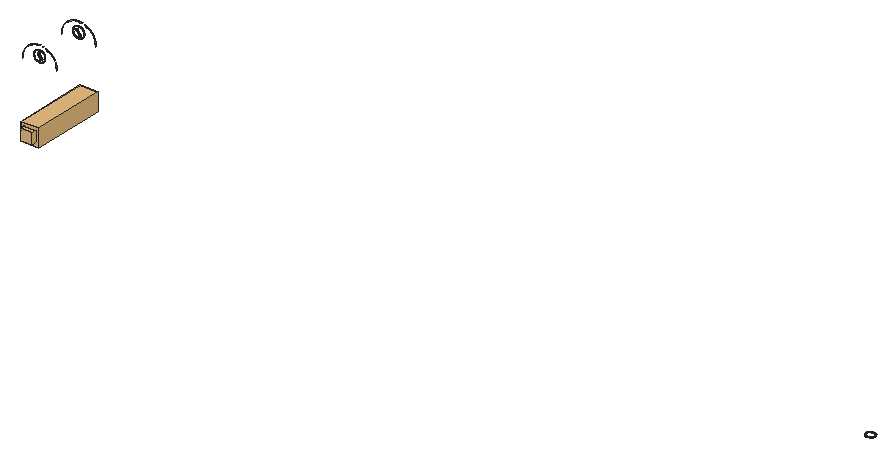
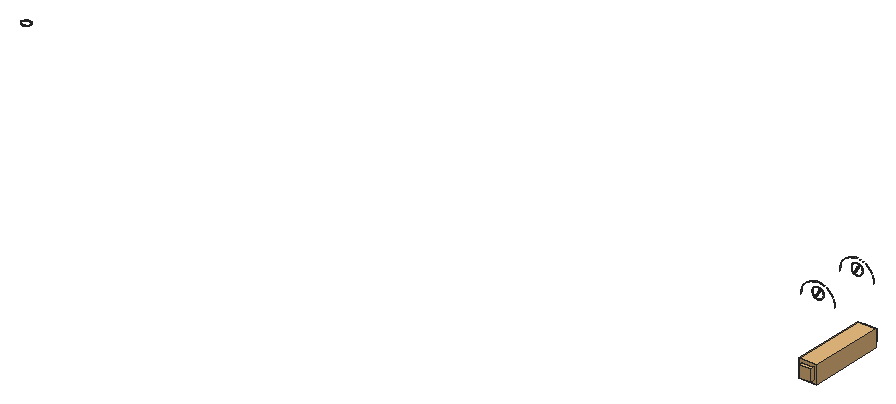
# SketchUp Ruby script. Lengths in inches.
U = 1.inch
M = Sketchup.active_model
def pt(a) = Geom::Point3d.new(a.map { |v| v * U })
def face(e, loops, mat)
  f = e.add_face(loops[0].map { |a| pt(a) })
  loops[1..].each { |l| e.add_face(l.map { |a| pt(a) }).erase! }
  f.material = f.back_material = mat if mat
  f
end
# faces: each face lists its corners as indices into pts; further lists are holes
def faces(e, pts, list, mat = nil) = list.each { |f| face(e, (f[0].is_a?(Array) ? f : [f]).map { |l| l.map { |i| pts[i] } }, mat) }
# xy, xz, yz: faces in a plane at the given z, y or x. An outline is a flat list of corners, or four numbers for a rectangle; further outlines are holes
def ring(l) = l.size == 4 ? [[l[0], l[1]], [l[2], l[1]], [l[2], l[3]], [l[0], l[3]]] : l.each_slice(2).to_a
def flat(e, list, mat, &to3) = list.each { |f| face(e, (f[0].is_a?(Array) ? f : [f]).map { |l| ring(l).map { |u, v| to3.(u, v) } }, mat) }
def xy(e, z, list, mat = nil) = flat(e, list, mat) { |x, y| [x, y, z] }
def xz(e, y, list, mat = nil) = flat(e, list, mat) { |x, z| [x, y, z] }
def yz(e, x, list, mat = nil) = flat(e, list, mat) { |y, z| [x, y, z] }
def lines(e, pts, list) = list.each { |a, b| e.add_line(pt(pts[a]), pt(pts[b])) }
# prism: a flat outline (further loops are holes) pulled along v
def prism(e, loops, v, mat = nil)
  f = face(e, loops, mat); d = Geom::Vector3d.new(v.map { |x| x * U })
  f.pushpull(f.normal.samedirection?(d) ? d.length : -d.length)
end
def box(e, o, s, mat = nil) = prism(e, [[o, [o[0] + s[0], o[1], o[2]], [o[0] + s[0], o[1] + s[1], o[2]], [o[0], o[1] + s[1], o[2]]]], [0, 0, s[2]], mat)
def at(x, y, z, deg = 0) = Geom::Transformation.translation(pt([x, y, z])) * Geom::Transformation.rotation(ORIGIN, Z_AXIS, deg.degrees)
def axes(o, x, y, z) = Geom::Transformation.new([*x, 0, *y, 0, *z, 0, *pt(o).to_a, 1])
def part(name) = M.definitions.add(name)
# library, detail: a bought-in or finely detailed component or shape, given as its bounding box
def library(name, o, s) = part(name).tap { |d| box(d.entities, o, s) }
def detail(e, o, s) = box(e.add_group.entities, o, s)
def put(e, d, t, mat = nil) = e.add_instance(d, t).tap { |i| i.material = mat if mat }
def group(e, t, mat = nil) = e.add_group.tap { |g| g.transformation = t; g.material = mat if mat }.entities
root = M.entities
M.materials.add("Material \#1").color = [140, 140, 140]
c1 = library("3DGeom~14_Defintion",[-102.17,352.37,-727.27],[204.35,204.35,1000])
c2 = library("3DGeom~1_Defintion",[-60.87,347.29,-704.08],[121.74,121.75,1000])
xy(root,193.77,[[371.53,115.15,371.46,115.17,371.53,115.17],[371.53,115.15,371.53,115.17,371.6,115.17],[371.53,115.15,371.6,115.17,371.6,115.15],[371.6,115.15,371.6,115.17,371.66,115.19],[371.6,115.15,371.66,115.19,371.67,115.17],
  [371.46,115.17,371.41,115.21,371.47,115.19],[371.46,115.17,371.47,115.19,371.53,115.17],[371.67,115.17,371.66,115.19,371.71,115.22],[371.67,115.17,371.71,115.22,371.72,115.21],[371.47,115.19,371.41,115.21,371.43,115.22],
  [371.41,115.21,371.375,115.26,371.43,115.22],[371.72,115.21,371.71,115.22,371.74,115.27],[371.72,115.21,371.74,115.27,371.76,115.26],[371.43,115.22,371.375,115.26,371.39,115.27],[371.375,115.26,371.36,115.32,371.39,115.27],
  [371.76,115.26,371.74,115.27,371.75,115.32],[371.76,115.26,371.75,115.32,371.77,115.32],[371.39,115.27,371.36,115.32,371.38,115.32],[371.36,115.32,371.375,115.38,371.38,115.32],[371.38,115.32,371.375,115.38,371.39,115.37],
  [371.75,115.32,371.74,115.37,371.77,115.32],[371.77,115.32,371.74,115.37,371.76,115.38],[371.39,115.37,371.375,115.38,371.41,115.43],[371.39,115.37,371.41,115.43,371.43,115.42],[371.74,115.37,371.71,115.42,371.76,115.38],
  [371.76,115.38,371.71,115.42,371.72,115.43],[371.43,115.42,371.41,115.43,371.46,115.47],[371.43,115.42,371.46,115.47,371.47,115.45],[371.71,115.42,371.66,115.45,371.72,115.43],[371.72,115.43,371.66,115.45,371.67,115.47],
  [371.47,115.45,371.46,115.47,371.53,115.49],[371.47,115.45,371.53,115.49,371.53,115.47],[371.66,115.45,371.6,115.47,371.67,115.47],[371.53,115.47,371.53,115.49,371.6,115.49],[371.53,115.47,371.6,115.49,371.6,115.47],
  [371.6,115.47,371.6,115.49,371.67,115.47]],"Material \#1")
xy(root,193.78,[[371.53,115.15,371.47,115.19,371.46,115.17],[371.53,115.15,371.53,115.17,371.47,115.19],[371.53,115.15,371.6,115.15,371.53,115.17],[371.6,115.15,371.6,115.17,371.53,115.17],[371.6,115.15,371.67,115.17,371.6,115.17],
  [371.46,115.17,371.43,115.22,371.41,115.21],[371.46,115.17,371.47,115.19,371.43,115.22],[371.6,115.17,371.67,115.17,371.66,115.19],[371.67,115.17,371.72,115.21,371.66,115.19],[371.66,115.19,371.72,115.21,371.71,115.22],
  [371.41,115.21,371.39,115.27,371.375,115.26],[371.41,115.21,371.43,115.22,371.39,115.27],[371.72,115.21,371.76,115.26,371.71,115.22],[371.71,115.22,371.76,115.26,371.74,115.27],[371.375,115.26,371.38,115.32,371.36,115.32],
  [371.375,115.26,371.39,115.27,371.38,115.32],[371.76,115.26,371.77,115.32,371.74,115.27],[371.74,115.27,371.77,115.32,371.75,115.32],[371.36,115.32,371.38,115.32,371.39,115.37],[371.36,115.32,371.39,115.37,371.375,115.38],
  [371.75,115.32,371.76,115.38,371.74,115.37],[371.75,115.32,371.77,115.32,371.76,115.38],[371.39,115.37,371.43,115.42,371.375,115.38],[371.74,115.37,371.72,115.43,371.71,115.42],[371.74,115.37,371.76,115.38,371.72,115.43],
  [371.375,115.38,371.43,115.42,371.41,115.43],[371.43,115.42,371.47,115.45,371.41,115.43],[371.71,115.42,371.67,115.47,371.66,115.45],[371.71,115.42,371.72,115.43,371.67,115.47],[371.41,115.43,371.47,115.45,371.46,115.47],
  [371.47,115.45,371.53,115.47,371.46,115.47],[371.66,115.45,371.6,115.49,371.6,115.47],[371.66,115.45,371.67,115.47,371.6,115.49],[371.46,115.47,371.53,115.47,371.53,115.49],[371.53,115.47,371.6,115.47,371.53,115.49],
  [371.6,115.47,371.6,115.49,371.53,115.49]],"Material \#1")
xz(root,114.63,[[337.35,195.92,337.36,196.05,337.36,195.92],[337.36,195.92,337.36,196.05,337.37,196.05],[338.75,195.92,338.74,196.05,338.77,195.92],[338.77,195.92,338.74,196.05,338.75,196.05],[338.06,195.97,338.01,195.98,338.06,195.99],
  [338.06,195.97,338.06,195.99,338.1,195.99],[338.06,195.97,338.1,195.99,338.1,195.98],[338.01,195.98,337.97,195.99,338.02,195.99],[338.01,195.98,338.02,195.99,338.06,195.99],[338.1,195.98,338.1,195.99,338.13,196],
  [338.1,195.98,338.13,196,338.14,195.99],[337.97,195.99,337.9375,196.01,337.98,196],[337.97,195.99,337.98,196,338.02,195.99],[338.14,195.99,338.13,196,338.17,196.02],[338.14,195.99,338.17,196.02,338.17,196.01],
  [337.98,196,337.9375,196.01,337.94,196.02],[337.9375,196.01,337.9,196.03,337.94,196.02],[338.17,196.01,338.17,196.02,338.2,196.04],[338.17,196.01,338.2,196.04,338.21,196.03],[337.94,196.02,337.9,196.03,337.91,196.04],
  [337.9,196.03,337.875,196.06,337.91,196.04],[338.21,196.03,338.2,196.04,338.23,196.0625],[338.21,196.03,338.23,196.0625,338.24,196.06],[337.91,196.04,337.875,196.06,337.88,196.0625],[337.36,196.05,337.39,196.17,337.37,196.05],
  [337.37,196.05,337.39,196.17,337.4,196.16],[338.74,196.05,338.71,196.16,338.75,196.05],[338.75,196.05,338.71,196.16,338.72,196.17],[337.875,196.06,337.85,196.09,337.88,196.0625],[338.24,196.06,338.23,196.0625,338.25,196.09],
  [338.24,196.06,338.25,196.09,338.26,196.09],[337.88,196.0625,337.85,196.09,337.86,196.09],[337.85,196.09,337.83,196.125,337.86,196.09],[337.86,196.09,337.83,196.125,337.85,196.13],[338.25,196.09,338.27,196.13,338.26,196.09],
  [338.26,196.09,338.27,196.13,338.28,196.125],[337.83,196.125,337.82,196.16,337.85,196.13],[338.28,196.125,338.27,196.13,338.28,196.16],[338.28,196.125,338.28,196.16,338.29,196.16],[337.85,196.13,337.82,196.16,337.84,196.16],
  [337.4,196.16,337.39,196.17,337.44,196.28],[337.4,196.16,337.44,196.28,337.45,196.27],[337.82,196.16,337.82,196.21,337.84,196.16],[337.84,196.16,337.82,196.21,337.83,196.21],[338.28,196.16,338.28,196.2,338.29,196.16],
  [338.29,196.16,338.28,196.2,338.29,196.2],[338.71,196.16,338.66,196.27,338.72,196.17],[338.72,196.17,338.66,196.27,338.67,196.28],[338.28,196.2,338.28,196.24,338.29,196.2],[338.29,196.2,338.28,196.24,338.29,196.24],
  [337.82,196.21,337.82,196.24,337.83,196.21],[337.83,196.21,337.82,196.24,337.84,196.24],[337.82,196.24,337.83,196.28,337.84,196.24],[337.84,196.24,337.83,196.28,337.85,196.28],[338.28,196.24,338.27,196.28,338.29,196.24],
  [338.29,196.24,338.27,196.28,338.28,196.28],[337.45,196.27,337.44,196.28,337.52,196.375],[337.45,196.27,337.52,196.375,337.52,196.37],[338.66,196.27,338.59,196.36,338.67,196.28],[337.83,196.28,337.85,196.32,337.85,196.28],
  [337.85,196.28,337.85,196.32,337.86,196.3125],[338.27,196.28,338.25,196.3125,338.28,196.28],[338.28,196.28,338.25,196.3125,338.26,196.32],[338.67,196.28,338.59,196.36,338.6,196.37],[337.86,196.3125,337.85,196.32,337.875,196.35],
  [337.86,196.3125,337.875,196.35,337.88,196.34],[338.25,196.3125,338.23,196.34,338.26,196.32],[338.26,196.32,338.23,196.34,338.24,196.35],[337.88,196.34,337.875,196.35,337.9,196.38],[337.88,196.34,337.9,196.38,337.91,196.37],
  [338.23,196.34,338.2,196.37,338.24,196.35],[338.24,196.35,338.2,196.37,338.21,196.38],[338.59,196.36,338.51,196.45,338.6,196.37],[337.52,196.37,337.52,196.375,337.6,196.46],[337.52,196.37,337.6,196.46,337.61,196.45],
  [337.91,196.37,337.9,196.38,337.9375,196.4],[337.91,196.37,337.9375,196.4,337.94,196.39],[338.2,196.37,338.17,196.39,338.21,196.38],[338.6,196.37,338.51,196.45,338.51,196.46],[338.21,196.38,338.17,196.39,338.17,196.4],
  [337.94,196.39,337.9375,196.4,337.97,196.42],[337.94,196.39,337.97,196.42,337.98,196.41],[338.17,196.39,338.13,196.41,338.17,196.4],[338.17,196.4,338.13,196.41,338.14,196.42],[337.98,196.41,337.97,196.42,338.01,196.43],
  [337.98,196.41,338.01,196.43,338.02,196.42],[338.13,196.41,338.1,196.42,338.14,196.42],[338.02,196.42,338.01,196.43,338.06,196.43],[338.02,196.42,338.06,196.43,338.06,196.42],[338.06,196.42,338.06,196.43,338.1,196.43],
  [338.06,196.42,338.1,196.43,338.1,196.42],[338.1,196.42,338.1,196.43,338.14,196.42],[337.61,196.45,337.6,196.46,337.7,196.52],[337.61,196.45,337.7,196.52,337.7,196.51],[338.51,196.45,338.41,196.51,338.51,196.46],
  [338.51,196.46,338.41,196.51,338.41,196.52],[337.7,196.51,337.7,196.52,337.81,196.57],[337.7,196.51,337.81,196.57,337.8125,196.5625],[338.41,196.51,338.3,196.5625,338.41,196.52],[338.41,196.52,338.3,196.5625,338.3,196.57],
  [337.8125,196.5625,337.81,196.57,337.93,196.61],[337.8125,196.5625,337.93,196.61,337.93,196.59],[338.3,196.5625,338.18,196.59,338.3,196.57],[338.3,196.57,338.18,196.59,338.18,196.61],[337.93,196.59,337.93,196.61,338.06,196.62],
  [337.93,196.59,338.06,196.62,338.06,196.61],[338.18,196.59,338.06,196.61,338.18,196.61],[338.06,196.61,338.06,196.62,338.18,196.61]],"Material \#1")
xz(root,116.63,[[337.35,195.92,337.36,195.92,337.36,196.05],[337.36,195.92,337.37,196.05,337.36,196.05],[338.75,195.92,338.77,195.92,338.74,196.05],[338.77,195.92,338.75,196.05,338.74,196.05],[338.06,195.97,338.06,195.99,338.01,195.98],
  [338.06,195.97,338.1,195.98,338.1,195.99],[338.06,195.97,338.1,195.99,338.06,195.99],[338.01,195.98,338.02,195.99,337.97,195.99],[338.01,195.98,338.06,195.99,338.02,195.99],[338.1,195.98,338.13,196,338.1,195.99],
  [338.1,195.98,338.14,195.99,338.13,196],[337.97,195.99,337.98,196,337.9375,196.01],[337.97,195.99,338.02,195.99,337.98,196],[338.14,195.99,338.17,196.02,338.13,196],[338.14,195.99,338.17,196.01,338.17,196.02],
  [337.98,196,337.94,196.02,337.9375,196.01],[337.9375,196.01,337.94,196.02,337.9,196.03],[338.17,196.01,338.2,196.04,338.17,196.02],[338.17,196.01,338.21,196.03,338.2,196.04],[337.94,196.02,337.91,196.04,337.9,196.03],
  [337.9,196.03,337.91,196.04,337.875,196.06],[338.21,196.03,338.23,196.0625,338.2,196.04],[338.21,196.03,338.24,196.06,338.23,196.0625],[337.91,196.04,337.88,196.0625,337.875,196.06],[337.36,196.05,337.37,196.05,337.39,196.17],
  [337.37,196.05,337.4,196.16,337.39,196.17],[338.74,196.05,338.75,196.05,338.71,196.16],[338.75,196.05,338.72,196.17,338.71,196.16],[337.875,196.06,337.88,196.0625,337.85,196.09],[338.24,196.06,338.25,196.09,338.23,196.0625],
  [338.24,196.06,338.26,196.09,338.25,196.09],[337.88,196.0625,337.86,196.09,337.85,196.09],[337.85,196.09,337.86,196.09,337.83,196.125],[337.86,196.09,337.85,196.13,337.83,196.125],[338.25,196.09,338.26,196.09,338.27,196.13],
  [338.26,196.09,338.28,196.125,338.27,196.13],[337.83,196.125,337.85,196.13,337.82,196.16],[338.28,196.125,338.28,196.16,338.27,196.13],[338.28,196.125,338.29,196.16,338.28,196.16],[337.85,196.13,337.84,196.16,337.82,196.16],
  [337.4,196.16,337.44,196.28,337.39,196.17],[337.4,196.16,337.45,196.27,337.44,196.28],[337.82,196.16,337.84,196.16,337.82,196.21],[337.84,196.16,337.83,196.21,337.82,196.21],[338.28,196.16,338.29,196.16,338.28,196.2],
  [338.29,196.16,338.29,196.2,338.28,196.2],[338.71,196.16,338.72,196.17,338.66,196.27],[338.72,196.17,338.67,196.28,338.66,196.27],[338.28,196.2,338.29,196.2,338.28,196.24],[338.29,196.2,338.29,196.24,338.28,196.24],
  [337.82,196.21,337.83,196.21,337.82,196.24],[337.83,196.21,337.84,196.24,337.82,196.24],[337.82,196.24,337.84,196.24,337.83,196.28],[337.84,196.24,337.85,196.28,337.83,196.28],[338.28,196.24,338.29,196.24,338.27,196.28],
  [338.29,196.24,338.28,196.28,338.27,196.28],[337.45,196.27,337.52,196.375,337.44,196.28],[337.45,196.27,337.52,196.37,337.52,196.375],[338.66,196.27,338.67,196.28,338.59,196.36],[337.83,196.28,337.85,196.28,337.85,196.32],
  [337.85,196.28,337.86,196.3125,337.85,196.32],[338.27,196.28,338.28,196.28,338.25,196.3125],[338.28,196.28,338.26,196.32,338.25,196.3125],[338.67,196.28,338.6,196.37,338.59,196.36],[337.86,196.3125,337.875,196.35,337.85,196.32],
  [337.86,196.3125,337.88,196.34,337.875,196.35],[338.25,196.3125,338.26,196.32,338.23,196.34],[338.26,196.32,338.24,196.35,338.23,196.34],[337.88,196.34,337.9,196.38,337.875,196.35],[337.88,196.34,337.91,196.37,337.9,196.38],
  [338.23,196.34,338.24,196.35,338.2,196.37],[338.24,196.35,338.21,196.38,338.2,196.37],[338.59,196.36,338.6,196.37,338.51,196.45],[337.52,196.37,337.6,196.46,337.52,196.375],[337.52,196.37,337.61,196.45,337.6,196.46],
  [337.91,196.37,337.9375,196.4,337.9,196.38],[337.91,196.37,337.94,196.39,337.9375,196.4],[338.2,196.37,338.21,196.38,338.17,196.39],[338.6,196.37,338.51,196.46,338.51,196.45],[338.21,196.38,338.17,196.4,338.17,196.39],
  [337.94,196.39,337.97,196.42,337.9375,196.4],[337.94,196.39,337.98,196.41,337.97,196.42],[338.17,196.39,338.17,196.4,338.13,196.41],[338.17,196.4,338.14,196.42,338.13,196.41],[337.98,196.41,338.01,196.43,337.97,196.42],
  [337.98,196.41,338.02,196.42,338.01,196.43],[338.13,196.41,338.14,196.42,338.1,196.42],[338.02,196.42,338.06,196.43,338.01,196.43],[338.02,196.42,338.06,196.42,338.06,196.43],[338.06,196.42,338.1,196.42,338.1,196.43],
  [338.06,196.42,338.1,196.43,338.06,196.43],[338.1,196.42,338.14,196.42,338.1,196.43],[337.61,196.45,337.7,196.52,337.6,196.46],[337.61,196.45,337.7,196.51,337.7,196.52],[338.51,196.45,338.51,196.46,338.41,196.51],
  [338.51,196.46,338.41,196.52,338.41,196.51],[337.7,196.51,337.81,196.57,337.7,196.52],[337.7,196.51,337.8125,196.5625,337.81,196.57],[338.41,196.51,338.41,196.52,338.3,196.5625],[338.41,196.52,338.3,196.57,338.3,196.5625],
  [337.8125,196.5625,337.93,196.61,337.81,196.57],[337.8125,196.5625,337.93,196.59,337.93,196.61],[338.3,196.5625,338.3,196.57,338.18,196.59],[338.3,196.57,338.18,196.61,338.18,196.59],[337.93,196.59,338.06,196.61,338.06,196.62],
  [337.93,196.59,338.06,196.62,337.93,196.61],[338.18,196.59,338.18,196.61,338.06,196.61],[338.06,196.61,338.18,196.61,338.06,196.62]],"Material \#1")
p = [[337.99,114.625,196.25],[337.99,114.65,196.25],[338.07,114.65,196.125],[338.07,114.625,196.125],[338.08,114.66,196.1],[338.08,114.63,196.1],
  [338.1,114.66,196.08],[338.1,114.64,196.08],[338.125,114.66,196.09],[338.125,114.64,196.09],[338.15,114.66,196.1],[338.15,114.64,196.1],
  [338.13,114.66,196.13],[338.13,114.63,196.13],[338.12,114.65,196.15],[338.12,114.625,196.15],[337.99,116.63,196.25],[338.07,116.63,196.125],
  [338.07,116.61,196.125],[337.99,116.61,196.25],[338.08,116.63,196.1],[338.08,116.6,196.1],[338.1,116.625,196.08],[338.1,116.6,196.08],
  [338.125,116.625,196.09],[338.125,116.6,196.09],[338.15,116.625,196.1],[338.15,116.6,196.1],[338.13,116.63,196.13],[338.13,116.6,196.13],
  [338.12,116.63,196.15],[338.12,116.61,196.15],[338.04,114.65,196.28],[338.04,114.625,196.28],[338.04,116.63,196.28],[338.04,116.61,196.28],
  [338.03,114.66,196.3],[338.03,114.63,196.3],[338.01,114.66,196.33],[338.01,114.64,196.33],[337.99,114.66,196.32],[337.99,114.64,196.32],
  [337.97,114.66,196.3],[337.97,114.64,196.3],[337.98,114.66,196.28],[337.98,114.63,196.28],[338.03,116.63,196.3],[338.03,116.6,196.3],
  [338.01,116.625,196.33],[338.01,116.6,196.33],[337.99,116.625,196.32],[337.99,116.6,196.32],[337.97,116.625,196.3],[337.97,116.6,196.3],
  [337.98,116.63,196.28],[337.98,116.6,196.28]]
faces(root,p,[[0,1,2],[2,3,0],[3,2,4],[4,5,3],[5,4,6],[6,7,5],[7,6,8],[8,9,7],
  [9,8,10],[10,11,9],[11,10,12],[12,13,11],[13,12,14],[14,15,13],[16,17,18],[18,19,16],
  [17,20,21],[21,18,17],[20,22,23],[23,21,20],[22,24,25],[25,23,22],[24,26,27],[27,25,24],
  [26,28,29],[29,27,26],[28,30,31],[31,29,28],[15,14,32],[32,33,15],[30,34,35],[35,31,30],
  [33,32,36],[36,37,33],[37,36,38],[38,39,37],[39,38,40],[40,41,39],[41,40,42],[42,43,41],
  [43,42,44],[44,45,43],[45,44,1],[1,0,45],[34,46,47],[47,35,34],[46,48,49],[49,47,46],
  [48,50,51],[51,49,48],[50,52,53],[53,51,50],[52,54,55],[55,53,52],[54,16,19],[19,55,54]],"Material \#1")
put(root,c1,axes([338.06,116.32,191.98],[0.00357,0,0],[0,0,0.00348],[0,0.00304,0]),"Material \#1")
put(root,c2,axes([338.06,116.32,191.98],[0.00398,0,0],[0,0,0.00387],[0,0.00338,0]),"Material \#1")
